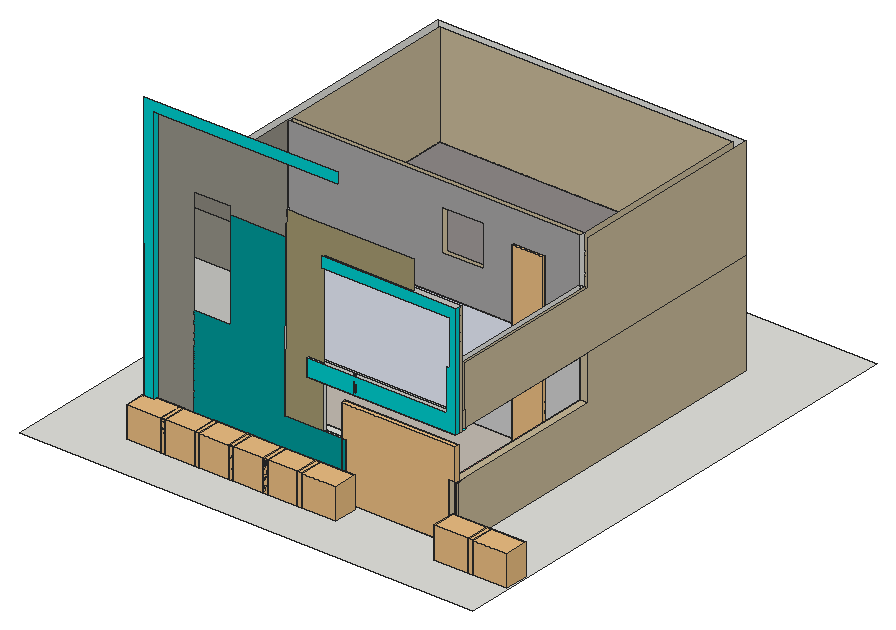
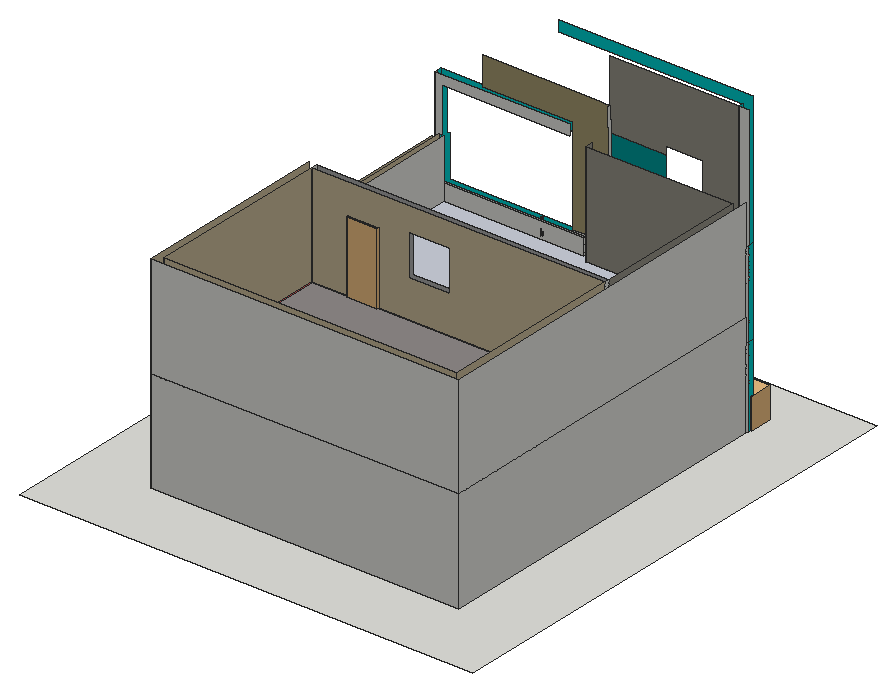
# SketchUp Ruby script. Lengths in inches.
U = 1.inch
M = Sketchup.active_model
def pt(a) = Geom::Point3d.new(a.map { |v| v * U })
def face(e, loops, mat)
  f = e.add_face(loops[0].map { |a| pt(a) })
  loops[1..].each { |l| e.add_face(l.map { |a| pt(a) }).erase! }
  f.material = f.back_material = mat if mat
  f
end
# faces: each face lists its corners as indices into pts; further lists are holes
def faces(e, pts, list, mat = nil) = list.each { |f| face(e, (f[0].is_a?(Array) ? f : [f]).map { |l| l.map { |i| pts[i] } }, mat) }
# xy, xz, yz: faces in a plane at the given z, y or x. An outline is a flat list of corners, or four numbers for a rectangle; further outlines are holes
def ring(l) = l.size == 4 ? [[l[0], l[1]], [l[2], l[1]], [l[2], l[3]], [l[0], l[3]]] : l.each_slice(2).to_a
def flat(e, list, mat, &to3) = list.each { |f| face(e, (f[0].is_a?(Array) ? f : [f]).map { |l| ring(l).map { |u, v| to3.(u, v) } }, mat) }
def xy(e, z, list, mat = nil) = flat(e, list, mat) { |x, y| [x, y, z] }
def xz(e, y, list, mat = nil) = flat(e, list, mat) { |x, z| [x, y, z] }
def yz(e, x, list, mat = nil) = flat(e, list, mat) { |y, z| [x, y, z] }
def lines(e, pts, list) = list.each { |a, b| e.add_line(pt(pts[a]), pt(pts[b])) }
# prism: a flat outline (further loops are holes) pulled along v
def prism(e, loops, v, mat = nil)
  f = face(e, loops, mat); d = Geom::Vector3d.new(v.map { |x| x * U })
  f.pushpull(f.normal.samedirection?(d) ? d.length : -d.length)
end
def box(e, o, s, mat = nil) = prism(e, [[o, [o[0] + s[0], o[1], o[2]], [o[0] + s[0], o[1] + s[1], o[2]], [o[0], o[1] + s[1], o[2]]]], [0, 0, s[2]], mat)
def at(x, y, z, deg = 0) = Geom::Transformation.translation(pt([x, y, z])) * Geom::Transformation.rotation(ORIGIN, Z_AXIS, deg.degrees)
def axes(o, x, y, z) = Geom::Transformation.new([*x, 0, *y, 0, *z, 0, *pt(o).to_a, 1])
def part(name) = M.definitions.add(name)
# library, detail: a bought-in or finely detailed component or shape, given as its bounding box
def library(name, o, s) = part(name).tap { |d| box(d.entities, o, s) }
def detail(e, o, s) = box(e.add_group.entities, o, s)
def put(e, d, t, mat = nil) = e.add_instance(d, t).tap { |i| i.material = mat if mat }
def group(e, t, mat = nil) = e.add_group.tap { |g| g.transformation = t; g.material = mat if mat }.entities
root = M.entities
M.materials.add("[Carrera Marble]").color = [207, 207, 207]
M.materials.add("[Color A02]").color = [255, 153, 153]
M.materials.add("[Color A03]").color = [255, 101, 101]
M.materials.add("[Color H05]").color = [0, 255, 255]
M.materials.add("[Color H06]").color = [0, 204, 204]
M.materials.add("[Color H07]").color = [0, 153, 153]
M.materials.add("[Field Rectangle Tile]").color = [196, 189, 179]
M.materials.add("[Formica Graystone]").color = [149, 146, 135]
M.materials.add("[Marble Carrara Floor Tile]").color = [204, 208, 219]
M.materials.add("[Quartz Light Brown]").color = [199, 184, 152]
M.materials.add("[Stone Marble]").color = [143, 138, 136]
M.materials.add("[Stone Vein Gray]").color = [166, 165, 165]
M.materials.add("[Translucent Glass Gray]1").color = [128, 128, 128]
M.materials["[Translucent Glass Gray]1"].alpha = 0.5
M.materials.add("[Wood Lumber ButtJoined]").color = [164, 152, 112]
c1 = library("DOOR (1)",[0,-8.5,0],[36,11.125,84])
c2 = library("plantas+internas",[0,0,0],[44.91,27.47,36.11])
c3 = library("gate",[-17.08,19.83,-10.33],[162.44,1,145.04])
c4 = part("Group\#7")
xy(c4.entities,0,[[0,0,32.48,1.97]])
xy(c4.entities,0.98,[[0.98,0,31.5,0.98],[0.98,0.98,31.5,1.97]])
xy(c4.entities,8.86,[[0.98,0,31.5,0.98],[0.98,0.98,31.5,1.97]])
xy(c4.entities,9.84,[[0,0,32.48,1.97]])
xz(c4.entities,0,[[[0,0,32.48,9.84],[0.98,0.98,31.5,8.86]]])
xz(c4.entities,0.98,[[0.98,0.98,31.5,8.86]],"[Translucent Glass Gray]1")
xz(c4.entities,1.97,[[[0,0,32.48,9.84],[0.98,0.98,31.5,8.86]]])
yz(c4.entities,0,[[0,0,1.97,9.84]])
yz(c4.entities,0.98,[[0,0.98,0.98,8.86],[0.98,0.98,1.97,8.86]])
yz(c4.entities,31.5,[[0,0.98,0.98,8.86],[0.98,0.98,1.97,8.86]])
yz(c4.entities,32.48,[[0,0,1.97,9.84]])
c5 = part("Group\#9")
xy(c5.entities,0,[[0,0,32.48,1.97]])
xy(c5.entities,0.98,[[0.98,0,31.5,0.98],[0.98,0.98,31.5,1.97]])
xy(c5.entities,71.85,[[0.98,0,31.5,0.98],[0.98,0.98,31.5,1.97]])
xy(c5.entities,72.83,[[0,0,32.48,1.97]])
xz(c5.entities,0,[[[0,0,32.48,72.83],[0.98,0.98,31.5,71.85]]])
xz(c5.entities,0.98,[[0.98,0.98,31.5,71.85]],"[Translucent Glass Gray]1")
xz(c5.entities,1.97,[[[0,0,32.48,72.83],[0.98,0.98,31.5,71.85]]])
yz(c5.entities,0,[[0,0,1.97,72.83]])
yz(c5.entities,0.98,[[0,0.98,0.98,71.85],[0.98,0.98,1.97,71.85]])
yz(c5.entities,31.5,[[0,0.98,0.98,71.85],[0.98,0.98,1.97,71.85]])
yz(c5.entities,32.48,[[0,0,1.97,72.83]])
c6 = part("FIXED+GLASS+WINDOW+WITH+TRANSOM")
g1 = group(c6.entities,at(0,0,0))
xy(g1,0,[[0,0,70.86,3.9375]])
xy(g1,1.97,[[1.97,0,34.45,0.98],[36.42,0,68.9,3.9375],[1.97,2.95,34.45,3.9375]])
xy(g1,86.61,[[1.97,0,34.45,3.9375],[34.45,0,36.42,3.9375],[36.42,0,68.9,3.9375]])
xy(g1,88.58,[[0,0,70.86,3.9375]])
xz(g1,0,[[[0,0,70.86,88.58],[1.97,1.97,34.45,86.61],[36.42,1.97,68.9,86.61]]])
xz(g1,3.9375,[[[0,0,70.86,88.58],[1.97,1.97,34.45,86.61],[36.42,1.97,68.9,86.61]]])
yz(g1,0,[[0,0,3.9375,88.58]])
yz(g1,1.97,[[0,1.97,3.9375,74.8],[0,76.77,3.9375,86.61]])
yz(g1,34.45,[[0,1.97,3.9375,86.61]])
yz(g1,36.42,[[0,1.97,3.9375,86.61]])
yz(g1,68.9,[[0,1.97,3.9375,86.61]])
yz(g1,70.86,[[0,0,3.9375,88.58]])
g2 = group(g1,at(1.97,0,74.8))
box(g2,[0,0,0],[66.93,3.9375,1.97])
put(g1,c4,at(1.97,0.98,76.77))
put(g1,c4,at(36.42,0.98,76.77))
put(g1,c5,at(1.97,0.98,1.97))
put(g1,c5,at(36.42,0.98,1.97))
xy(root,0,[[[0,0,528.77,588.77],[84.38,75.38,84.38,504.38,444.38,504.38,444.38,84.38,444.32,84.38,444.32,81.38,435.38,81.38,435.38,93.38,314.97,93.38,314.97,75.38]],[84.38,75.38,95.53,81.38],[95.53,75.38,314.97,81.38],[84.38,81.38,243.82,84.38],[243.82,81.38,314.97,84.38],
  [435.38,81.38,444.32,84.38],[84.38,84.38,84.38,504.38,444.38,504.38,444.38,84.38,435.38,84.38,435.38,495.38,93.38,495.38,93.38,93.38,314.97,93.38,314.97,84.38],[93.38,273.125,357.88,279.65],[393.88,273.125,435.38,279.65]])
xy(root,0,[[93.38,93.38,435.38,93.38,435.38,273.125,393.88,273.125,393.88,279.65,357.88,279.65,357.88,273.125,93.38,273.125]],"[Field Rectangle Tile]")
xy(root,0,[[93.38,279.65,435.38,495.38]],"[Stone Marble]")
xy(root,15.14,[[95.53,75.38,314.97,81.38]],"[Color H06]")
xy(root,44.61,[[274.3,273.125,322.3,279.65]])
xy(root,67.6875,[[264.38,84.38,314.97,93.38]])
xy(root,67.75,[[243.82,81.38,288.89,84.38],[288.89,81.38,314.97,84.38]])
xy(root,68,[[435.38,81.38,444.38,273.125]],"[Quartz Light Brown]")
xy(root,84,[[357.88,273.125,393.88,279.65]])
xy(root,92.61,[[274.3,273.125,322.3,279.65]])
xy(root,120,[[325.24,81.02,324.97,81.06,324.71,81.16,324.49,81.33,324.32,81.55,324.22,81.81,324.18,82.08,324.22,82.36,324.32,82.61,324.49,82.83,324.71,83,324.97,83.11,325.24,83.15,325.52,83.11,325.77,83,325.99,82.83,326.16,82.61,326.27,82.36,326.31,82.08,326.27,81.81,326.16,81.55,325.99,81.33,325.77,81.16,325.52,81.06],[272.14,81.38,288.89,84.38],[84.38,84.38,84.38,504.38,444.38,504.38,444.38,273.125,435.38,273.125,435.38,495.38,93.38,495.38,93.38,93.38,264.38,93.38,264.38,84.38],[272.14,84.38,435.38,86.51],[93.38,273.125,357.88,279.65],
  [393.88,273.125,435.38,279.65]])
xy(root,120,[[[272.14,78.76,272.14,81.38,288.89,81.38,288.89,84.38,435.38,84.38,435.38,78.76],[325.24,81.02,325.52,81.06,325.77,81.16,325.99,81.33,326.16,81.55,326.27,81.81,326.31,82.08,326.27,82.36,326.16,82.61,325.99,82.83,325.77,83,325.52,83.11,325.24,83.15,324.97,83.11,324.71,83,324.49,82.83,324.32,82.61,324.22,82.36,324.18,82.08,324.22,81.81,324.32,81.55,324.49,81.33,324.71,81.16,324.97,81.06]],[435.38,78.76,444.38,84.38],[444.38,78.76,445.9,84.38],[435.38,84.38,441.2,86.51],[441.2,84.38,444.38,86.51],
  [444.38,84.38,445.9,86.51],[435.38,86.51,441.2,273.125],[441.2,86.51,444.38,273.125],[444.38,86.51,445.9,93.38]],"[Color H05]")
xy(root,120,[[357.88,273.125,393.88,279.65]],"[Formica Graystone]")
xy(root,120,[[264.38,84.38,272.14,84.38,272.14,86.51,435.38,86.51,435.38,273.125,93.38,273.125,93.38,93.38,264.38,93.38]],"[Marble Carrara Floor Tile]")
xy(root,120,[[93.38,279.65,435.38,495.38]],"[Stone Marble]")
xz(root,75.38,[[84.38,0,314.97,0,314.97,15.14,95.53,15.14,95.53,336.625,310.04,336.625,310.04,348.625,84.38,348.625]],"[Color H06]")
xz(root,78.76,[[272.14,120,445.9,120,445.9,252,288.89,252,288.89,240,438.6,240,438.6,188,435.38,188,435.38,139.375,272.14,139.375]],"[Color H06]")
xz(root,81.38,[[84.38,0,95.53,336.625],[95.53,0,243.82,15.14],[272.14,120,288.89,123.625],[272.14,123.625,288.89,131.375],[272.14,131.375,288.89,139.375]])
xz(root,81.38,[[137.82,15.14,314.97,15.14,314.97,67.75,243.82,67.75,245.39,255.81,180.63,255.81,180.63,141.25,137.82,141.25]],"[Color H07]")
xz(root,81.38,[[95.53,15.14,137.82,15.14,137.82,264.8125,180.63,264.8125,180.63,255.81,245.39,255.81,245.63,284.5,245.63,336.625,95.53,336.625]],"[Formica Graystone]")
xz(root,81.38,[[435.38,0,444.32,0,444.32,67.6875,444.38,67.6875,444.38,68,435.38,68]],"[Quartz Light Brown]")
xz(root,81.38,[[243.82,67.75,288.89,67.75,288.89,120,272.14,120,272.14,139.375,288.89,139.375,288.89,252,394.7,252,394.7,284.625,264.38,284.625,264.38,284.5,245.63,284.5,245.39,255.81]],"[Wood Lumber ButtJoined]")
xz(root,84.38,[[84.38,0,243.82,93.4375],[444.32,0,444.38,67.6875],[264.38,67.6875,288.89,67.75],[288.89,67.6875,314.97,67.75],[243.82,67.75,243.82,120,244.26,120],
  [243.82,67.75,264.38,67.75,264.38,120,244.26,120],[264.38,67.75,288.89,120],[84.38,93.4375,243.82,120],[84.38,120,243.82,194.4375],[243.82,120,243.82,139.375,244.42,139.375,244.26,120],
  [244.26,120,264.38,120,264.38,139.375,244.42,139.375],[264.38,120,272.14,139.375],[272.14,120,435.38,139.375],[435.38,120,438.6,123.625],[438.6,120,441.2,123.625],
  [441.2,120,444.38,133.25],[435.38,123.625,438.6,131.375],[438.6,123.625,441.2,131.375],[435.38,131.375,438.6,133.25],[438.6,131.375,441.2,133.25],
  [435.38,133.25,438.6,139.375],[438.6,133.25,441.2,139.375],[441.2,133.25,444.38,139.375]])
xz(root,86.51,[[272.14,120,272.14,139.375,441.2,139.375,441.2,188,438.6,188,438.6,240,288.89,240,288.89,252,445.9,252,445.9,120]])
xz(root,93.38,[[93.38,0,93.38,120,264.38,120,264.38,67.6875,314.97,67.6875,314.97,0]],"[Color A02]")
xz(root,93.38,[[93.38,120,264.38,240]],"[Formica Graystone]")
xz(root,273.125,[[435.38,120,441.2,188]])
xz(root,273.125,[[[93.38,0,357.88,0,357.88,84,393.88,84,393.88,0,435.38,0,435.38,120,93.38,120],[274.3,44.61,322.3,92.61]]],"[Carrera Marble]")
xz(root,273.125,[[435.38,68,444.38,120]],"[Quartz Light Brown]")
xz(root,273.125,[[[93.38,120,357.88,120,357.88,204,393.88,204,393.88,120,435.38,120,435.38,240,93.38,240],[274.3,164.61,322.3,212.61]]],"[Stone Vein Gray]")
xz(root,279.65,[[[93.38,0,93.38,120,435.38,120,435.38,0,393.88,0,393.88,84,357.88,84,357.88,0],[274.3,44.61,322.3,92.61]]],"[Formica Graystone]")
xz(root,279.65,[[[93.38,120,93.38,240,435.38,240,435.38,120,393.88,120,393.88,204,357.88,204,357.88,120],[274.3,164.61,322.3,212.61]]],"[Quartz Light Brown]")
xz(root,495.38,[[93.38,0,435.38,120]],"[Formica Graystone]")
xz(root,495.38,[[93.38,120,435.38,240]],"[Quartz Light Brown]")
xz(root,504.38,[[84.38,0,444.38,120],[84.38,120,444.38,240]])
yz(root,84.38,[[81.38,0,84.38,93.4375],[84.38,0,504.38,120],[81.38,93.4375,84.38,194.4375],[84.38,120,504.38,240]])
yz(root,84.38,[[75.38,0,81.38,93.4375],[75.38,93.4375,81.38,194.4375]],"[Color H06]")
yz(root,93.38,[[273.125,0,279.65,120],[273.125,120,279.65,240]])
yz(root,93.38,[[93.38,0,273.125,120]],"[Color A02]")
yz(root,93.38,[[279.65,0,495.38,120],[93.38,120,273.125,240]],"[Formica Graystone]")
yz(root,93.38,[[279.65,120,495.38,240]],"[Quartz Light Brown]")
yz(root,95.53,[[75.38,15.14,81.38,336.625]],"[Color H06]")
yz(root,264.38,[[84.38,67.6875,93.38,120]])
yz(root,264.38,[[84.38,120,93.38,240]],"[Formica Graystone]")
yz(root,272.14,[[78.76,120,81.38,123.625],[81.38,120,84.38,123.625],[84.38,120,86.51,123.625],[78.76,123.625,81.38,131.375],[81.38,123.625,84.38,131.375],
  [84.38,123.625,86.51,131.375],[78.76,131.375,81.38,139.375],[81.38,131.375,84.38,139.375],[84.38,131.375,86.51,139.375]])
yz(root,274.3,[[273.125,44.61,279.65,92.61]])
yz(root,288.89,[[81.38,67.75,84.38,120]])
yz(root,314.97,[[75.38,0,93.38,0,93.38,67.6875,84.38,67.6875,84.38,67.75,81.38,67.75,81.38,15.14,75.38,15.14]],"[Color H06]")
yz(root,322.3,[[273.125,44.61,279.65,92.61]])
yz(root,357.88,[[273.125,0,279.65,84]])
yz(root,357.88,[[273.125,120,279.65,204]],"[Formica Graystone]")
yz(root,393.88,[[273.125,0,279.65,84]])
yz(root,393.88,[[273.125,120,279.65,204]],"[Formica Graystone]")
yz(root,435.38,[[273.125,0,279.65,120],[84.38,120,84.38,139.375,86.51,139.375,86.51,188,273.125,188,273.125,120],[273.125,120,279.65,240]])
yz(root,435.38,[[81.38,0,273.125,68]],"[Color A02]")
yz(root,435.38,[[279.65,0,495.38,120]],"[Color A03]")
yz(root,435.38,[[279.65,120,495.38,240]],"[Quartz Light Brown]")
yz(root,441.2,[[84.38,120,273.125,120,273.125,188,86.51,188,86.51,139.375,84.38,139.375]],"[Quartz Light Brown]")
yz(root,444.32,[[81.38,0,84.38,67.75]],"[Quartz Light Brown]")
yz(root,444.38,[[81.38,67.6875,81.45,68],[81.45,67.6875,84.01,68],[84.01,67.6875,93.38,68]])
yz(root,444.38,[[84.38,0,504.38,0,504.38,120,273.125,120,273.125,68,93.38,68,93.38,67.6875,84.38,67.6875],[84.38,120,93.38,139.375],[93.38,120,504.38,120,504.38,240,273.125,240,273.125,188,93.38,188]],"[Quartz Light Brown]")
yz(root,445.9,[[78.76,120,84.38,252]],"[Color H06]")
yz(root,445.9,[[84.38,120,86.51,252]],"[Quartz Light Brown]")
p = [[245.63,81.38,284.5],[245.39,81.38,255.81],[243.82,81.38,67.75],[243.82,84.38,67.75],[244.26,84.38,120],[244.42,84.38,139.375],
  [245.26,84.38,240],[245.63,84.38,284.5],[325.24,81.02,139.375],[324.97,81.06,139.375],[324.97,81.06,120],[325.24,81.02,120],
  [325.52,81.06,139.375],[325.52,81.06,120],[324.71,81.16,139.375],[324.71,81.16,120],[325.77,81.16,139.375],[325.77,81.16,120],
  [324.49,81.33,139.375],[324.49,81.33,120],[325.99,81.33,139.375],[325.99,81.33,120],[324.32,81.55,139.375],[324.32,81.55,120],
  [326.16,81.55,139.375],[326.16,81.55,120],[324.22,81.81,139.375],[324.22,81.81,120],[326.27,81.81,139.375],[326.27,81.81,120],
  [324.18,82.08,139.375],[324.18,82.08,120],[326.31,82.08,139.375],[326.31,82.08,120],[324.22,82.36,139.375],[324.22,82.36,120],
  [326.27,82.36,139.375],[326.27,82.36,120],[324.32,82.61,139.375],[324.32,82.61,120],[326.16,82.61,139.375],[326.16,82.61,120],
  [324.49,82.83,139.375],[324.49,82.83,120],[325.99,82.83,139.375],[325.99,82.83,120],[324.71,83,139.375],[324.71,83,120],
  [325.77,83,139.375],[325.77,83,120],[324.97,83.11,139.375],[324.97,83.11,120],[325.52,83.11,139.375],[325.52,83.11,120],
  [325.24,83.15,139.375],[325.24,83.15,120],[435.38,78.76,133.25],[435.38,84.38,133.25],[444.38,78.76,133.25],[444.38,84.38,133.25],
  [435.38,78.76,123.625],[435.38,84.38,123.625],[288.89,81.38,123.625],[288.89,84.38,123.625],[435.38,78.76,131.375],[435.38,84.38,131.375],
  [288.89,81.38,131.375],[288.89,84.38,131.375],[243.82,84.38,93.4375],[243.82,81.38,93.4375],[137.82,79.38,0],[314.97,81.38,0],
  [314.97,84.38,67.75],[314.97,93.38,67.75],[444.32,84.38,67.6875],[435.38,84.38,67.6875],[435.38,93.38,67.6875],[444.38,93.38,67.6875],
  [435.38,84.01,67.6875],[444.38,84.01,67.6875]]
faces(root,p,[[0,1,2,3,4,5,6,7],[8,9,10,11],[12,8,11,13],[9,14,15,10],[16,12,13,17],[14,18,19,15],[20,16,17,21],[18,22,23,19],
  [24,20,21,25],[22,26,27,23],[28,24,25,29],[26,30,31,27],[32,28,29,33],[30,34,35,31],[36,32,33,37],[34,38,39,35],
  [40,36,37,41],[38,42,43,39],[44,40,41,45],[42,46,47,43],[48,44,45,49],[46,50,51,47],[52,48,49,53],[50,54,55,51],
  [54,52,53,55]])
lines(root,p,[[56,57],[58,59],[60,61],[62,63],[64,65],[66,67],[68,69],[70,71],[72,73],[74,75],[76,77],[78,79]])
put(root,c1,at(357.88,279,0))
put(root,c2,at(82.67,51.44,0))
put(root,c2,at(122.61,51.44,0))
put(root,c2,at(162.55,51.44,0))
put(root,c2,at(202.49,51.44,0))
put(root,c2,at(242.42,51.44,0))
put(root,c2,at(282.36,51.44,0))
put(root,c2,at(442.11,51.44,0))
put(root,c2,at(482.05,51.44,0))
put(root,c3,axes([323.84,191.01,9.42],[0.81889,0,0],[0,-5.26282,0],[0,0,0.70981]))
put(root,c6,axes([274.3,272.5,44.61],[0.68379,0,0],[0,0.54286,0],[0,0,0.54286]))
put(root,c1,at(357.63,279,120))
